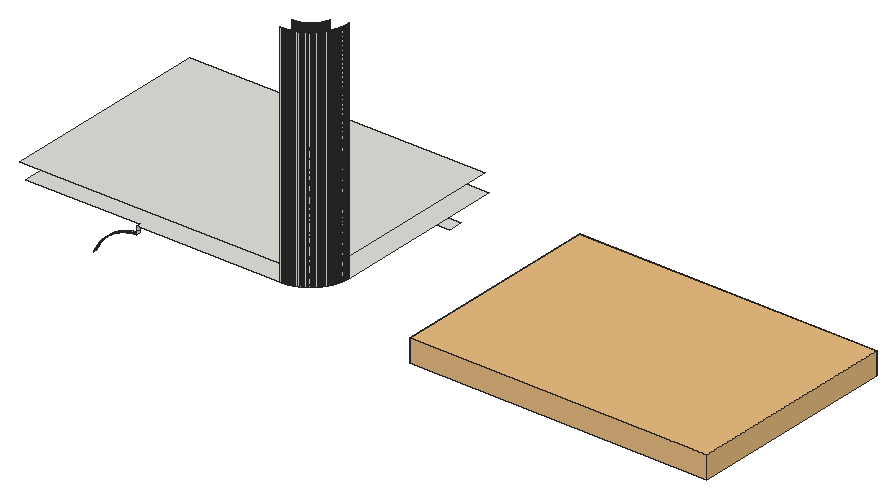
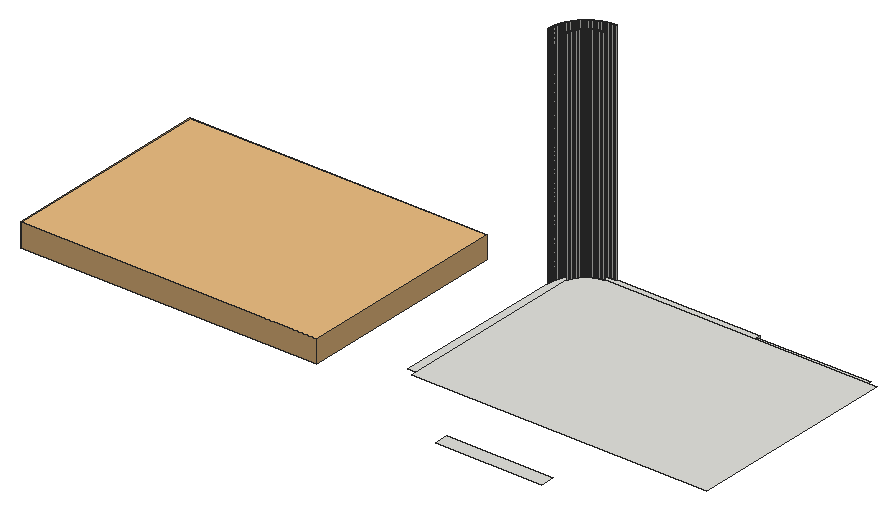
# SketchUp Ruby script. Lengths in inches.
U = 1.inch
M = Sketchup.active_model
def pt(a) = Geom::Point3d.new(a.map { |v| v * U })
def face(e, loops, mat)
  f = e.add_face(loops[0].map { |a| pt(a) })
  loops[1..].each { |l| e.add_face(l.map { |a| pt(a) }).erase! }
  f.material = f.back_material = mat if mat
  f
end
# faces: each face lists its corners as indices into pts; further lists are holes
def faces(e, pts, list, mat = nil) = list.each { |f| face(e, (f[0].is_a?(Array) ? f : [f]).map { |l| l.map { |i| pts[i] } }, mat) }
# xy, xz, yz: faces in a plane at the given z, y or x. An outline is a flat list of corners, or four numbers for a rectangle; further outlines are holes
def ring(l) = l.size == 4 ? [[l[0], l[1]], [l[2], l[1]], [l[2], l[3]], [l[0], l[3]]] : l.each_slice(2).to_a
def flat(e, list, mat, &to3) = list.each { |f| face(e, (f[0].is_a?(Array) ? f : [f]).map { |l| ring(l).map { |u, v| to3.(u, v) } }, mat) }
def xy(e, z, list, mat = nil) = flat(e, list, mat) { |x, y| [x, y, z] }
def xz(e, y, list, mat = nil) = flat(e, list, mat) { |x, z| [x, y, z] }
def yz(e, x, list, mat = nil) = flat(e, list, mat) { |y, z| [x, y, z] }
def lines(e, pts, list) = list.each { |a, b| e.add_line(pt(pts[a]), pt(pts[b])) }
# prism: a flat outline (further loops are holes) pulled along v
def prism(e, loops, v, mat = nil)
  f = face(e, loops, mat); d = Geom::Vector3d.new(v.map { |x| x * U })
  f.pushpull(f.normal.samedirection?(d) ? d.length : -d.length)
end
def box(e, o, s, mat = nil) = prism(e, [[o, [o[0] + s[0], o[1], o[2]], [o[0] + s[0], o[1] + s[1], o[2]], [o[0], o[1] + s[1], o[2]]]], [0, 0, s[2]], mat)
def at(x, y, z, deg = 0) = Geom::Transformation.translation(pt([x, y, z])) * Geom::Transformation.rotation(ORIGIN, Z_AXIS, deg.degrees)
def axes(o, x, y, z) = Geom::Transformation.new([*x, 0, *y, 0, *z, 0, *pt(o).to_a, 1])
def part(name) = M.definitions.add(name)
# library, detail: a bought-in or finely detailed component or shape, given as its bounding box
def library(name, o, s) = part(name).tap { |d| box(d.entities, o, s) }
def detail(e, o, s) = box(e.add_group.entities, o, s)
def put(e, d, t, mat = nil) = e.add_instance(d, t).tap { |i| i.material = mat if mat }
def group(e, t, mat = nil) = e.add_group.tap { |g| g.transformation = t; g.material = mat if mat }.entities
root = M.entities
c1 = library("Group\#26",[0,0,-14.0625],[184.56,132,14.0625])
xy(root,222,[[224.45,276,290.45,285]])
xy(root,251,[[201.56,144,201.56,146,131,146,131,276,314.45,276,314.45,167.375,314.43,167.06,314.42,166.75,314.4,166.43,314.38,166.12,314.35,165.81,314.32,165.49,314.29,165.18,314.21,164.56,314.16,164.25,314.11,163.9375,314.05,163.63,313.93,163.01,313.86,162.71,313.79,162.4,313.71,162.09,313.64,161.79,313.55,161.49,313.47,161.1875,313.375,160.89,313.28,160.59,313.08,159.99,312.97,159.7,312.86,159.4,312.74,159.11,312.625,158.82,312.5,158.53,312.38,158.24,312.25,157.95,312.12,157.67,311.84,157.11,311.69,156.83,311.55,156.55,311.39,156.28,311.24,156,310.92,155.46,310.75,155.2,310.58,154.93,310.41,154.67,310.05,154.15,309.87,153.9,309.68,153.64,309.3,153.14,309.1,152.9,308.91,152.66,308.7,152.42,308.5,152.18,308.29,151.94,308.08,151.71,307.86,151.48,307.64,151.26,307.42,151.03,307.2,150.8125,306.97,150.59,306.28,149.96,306.04,149.75,305.56,149.35,305.3125,149.15,304.8125,148.77,304.56,148.59,304.3,148.4,304.05,148.22,303.79,148.05,303.52,147.875,303.26,147.7,302.99,147.54,302.72,147.375,302.45,147.22,302.18,147.0625,301.91,146.91,301.63,146.76,300.79,146.34,300.5,146.21,300.22,146.08,299.93,145.95,299.35,145.71,299.05,145.6,298.76,145.49,298.46,145.38,298.17,145.28,297.57,145.08,296.97,144.9,296.67,144.82,296.36,144.74,296.06,144.67,295.75,144.59,295.44,144.53,295.14,144.46,294.83,144.4,293.9,144.25,293.59,144.21,293.27,144.17,292.96,144.13,292.65,144.1,292.34,144.08,292.02,144.05,291.71,144.03,291.4,144.02,291.08,144.01,290.77,144]])
xy(root,254.81,[[122,153,290.65,153,290.85,153.01,291.04,153.01,291.24,153.02,291.43,153.03,291.63,153.05,291.83,153.06,292.02,153.08,292.22,153.11,292.41,153.13,292.61,153.16,292.8,153.1875,292.99,153.22,293.1875,153.25,293.38,153.29,293.76,153.37,293.96,153.42,294.15,153.46,294.34,153.51,294.53,153.57,294.71,153.62,295.09,153.74,295.27,153.8,295.46,153.86,295.65,153.93,296.19,154.14,296.375,154.22,296.55,154.3,296.91,154.46,297.09,154.55,297.26,154.64,297.4375,154.73,297.61,154.82,297.78,154.91,298.29,155.21,298.46,155.32,298.62,155.42,298.79,155.53,299.11,155.75,299.27,155.87,299.43,155.98,299.58,156.1,299.74,156.22,299.89,156.34,300.04,156.47,300.2,156.6,300.34,156.72,300.49,156.85,300.64,156.99,300.78,157.12,301.2,157.54,301.33,157.68,301.47,157.82,301.6,157.97,301.73,158.11,301.99,158.41,302.11,158.5625,302.23,158.72,302.35,158.87,302.59,159.19,302.7,159.34,302.82,159.51,302.93,159.67,303.03,159.83,303.14,160,303.24,160.16,303.64,160.84,303.73,161.02,303.82,161.19,303.91,161.37,303.99,161.54,304.08,161.72,304.24,162.08,304.3125,162.26,304.39,162.44,304.53,162.81,304.59,162.99,304.66,163.18,304.72,163.37,304.78,163.55,304.84,163.74,304.99,164.31,305,164.34,305,285,122,285]])
xz(root,144,[[290.45,251,290.77,392.81]])
xz(root,153,[[290.45,254.81,290.65,392.81]])
xz(root,153.01,[[290.85,254.81,291.04,392.81]])
yz(root,201.56,[[144,248,146,251]])
yz(root,314.45,[[167.375,251,167.6875,392.81],[167.6875,251,168,392.81]])
p = [[175.15,144,227.49],[175.01,144,227.16],[175.01,146,227.16],[175.15,146,227.49],[175.3,144,227.82],[175.3,146,227.82],
  [175.44,144,228.14],[175.44,146,228.14],[175.59,144,228.47],[175.59,146,228.47],[175.74,144,228.79],[175.74,146,228.79],
  [175.9,144,229.11],[175.9,146,229.11],[176.06,144,229.42],[176.06,146,229.42],[176.22,144,229.74],[176.22,146,229.74],
  [176.39,144,230.05],[176.39,146,230.05],[176.5625,144,230.36],[176.5625,146,230.36],[176.74,144,230.67],[176.74,146,230.67],
  [176.92,144,230.98],[176.92,146,230.98],[177.1,144,231.29],[177.1,146,231.29],[177.28,144,231.59],[177.28,146,231.59],
  [177.47,144,231.89],[177.47,146,231.89],[177.66,144,232.19],[177.66,146,232.19],[177.86,144,232.49],[177.86,146,232.49],
  [178.06,144,232.78],[178.06,146,232.78],[178.26,144,233.07],[178.26,146,233.07],[178.47,144,233.36],[178.47,146,233.36],
  [178.68,144,233.65],[178.68,146,233.65],[178.89,144,233.9375],[178.89,146,233.9375],[179.1,144,234.22],[179.1,146,234.22],
  [179.32,144,234.5],[179.32,146,234.5],[179.55,144,234.78],[179.55,146,234.78],[179.77,144,235.05],[179.77,146,235.05],
  [180,144,235.33],[180,146,235.33],[180.23,144,235.6],[180.23,146,235.6],[180.46,144,235.86],[180.46,146,235.86],
  [180.7,144,236.13],[180.7,146,236.13],[180.94,144,236.39],[180.94,146,236.39],[181.1875,144,236.65],[181.1875,146,236.65],
  [181.43,144,236.9],[181.43,146,236.9],[181.68,144,237.16],[181.68,146,237.16],[181.93,144,237.41],[181.93,146,237.41],
  [182.19,144,237.66],[182.19,146,237.66],[182.45,144,237.9],[182.45,146,237.9],[182.71,144,238.14],[182.71,146,238.14],
  [182.97,144,238.38],[182.97,146,238.38],[183.24,144,238.62],[183.24,146,238.62],[183.51,144,238.85],[183.51,146,238.85],
  [183.78,144,239.08],[183.78,146,239.08],[184.05,144,239.31],[184.05,146,239.31],[184.33,144,239.53],[184.33,146,239.53],
  [184.61,144,239.75],[184.61,146,239.75],[184.89,144,239.97],[184.89,146,239.97],[185.18,144,240.18],[185.18,146,240.18],
  [185.46,144,240.39],[185.46,146,240.39],[185.75,144,240.6],[185.75,146,240.6],[186.04,144,240.8],[186.04,146,240.8],
  [186.34,144,241],[186.34,146,241],[186.63,144,241.2],[186.63,146,241.2],[186.93,144,241.39],[186.93,146,241.39],
  [187.23,144,241.58],[187.23,146,241.58],[187.54,144,241.77],[187.54,146,241.77],[187.84,144,241.95],[187.84,146,241.95],
  [188.15,144,242.13],[188.15,146,242.13],[188.46,144,242.31],[188.46,146,242.31],[188.77,144,242.48],[188.77,146,242.48],
  [189.08,144,242.65],[189.08,146,242.65],[189.4,144,242.8125],[189.4,146,242.8125],[189.71,144,242.97],[189.71,146,242.97],
  [190.03,144,243.13],[190.03,146,243.13],[190.35,144,243.29],[190.35,146,243.29],[190.67,144,243.4375],[190.67,146,243.4375],
  [191,144,243.58],[191,146,243.58],[191.32,144,243.73],[191.32,146,243.73],[191.65,144,243.87],[191.65,146,243.87],
  [191.98,144,244],[191.98,146,244],[192.31,144,244.13],[192.31,146,244.13],[192.64,144,244.26],[192.64,146,244.26],
  [192.97,144,244.39],[192.97,146,244.39],[193.31,144,244.51],[193.31,146,244.51],[193.64,144,244.625],[193.64,146,244.625],
  [193.98,144,244.74],[193.98,146,244.74],[194.32,144,244.85],[194.32,146,244.85],[194.66,144,244.95],[194.66,146,244.95],
  [195,144,245.05],[195,146,245.05],[195.34,144,245.15],[195.34,146,245.15],[195.68,144,245.24],[195.68,146,245.24],
  [196.03,144,245.33],[196.03,146,245.33],[196.375,144,245.42],[196.375,146,245.42],[196.72,144,245.5],[196.72,146,245.5],
  [197.07,144,245.58],[197.07,146,245.58],[197.42,144,245.65],[197.42,146,245.65],[197.76,144,245.72],[197.76,146,245.72],
  [198.11,144,245.78],[198.11,146,245.78],[198.46,144,245.85],[198.46,146,245.85],[198.81,144,245.9],[198.81,146,245.9],
  [199.17,144,245.96],[199.17,146,245.96],[199.52,144,246.01],[199.52,146,246.01],[199.87,144,246.05],[199.87,146,246.05],
  [200.22,144,246.09],[200.22,146,246.09],[200.58,144,246.13],[200.58,146,246.13],[200.93,144,246.16],[200.93,146,246.16],
  [201.29,144,246.19],[201.29,146,246.19],[201.64,144,246.22],[201.64,146,246.22],[201.56,144,248],[201.56,146,248],
  [290.77,144,392.81],[290.77,144,251],[291.08,144.01,251],[291.08,144.01,392.81],[291.4,144.02,251],[291.4,144.02,392.81],
  [291.71,144.03,251],[291.71,144.03,392.81],[292.02,144.05,251],[292.02,144.05,392.81],[292.34,144.08,251],[292.34,144.08,392.81],
  [292.65,144.1,251],[292.65,144.1,392.81],[292.96,144.13,251],[292.96,144.13,392.81],[293.27,144.17,251],[293.27,144.17,392.81],
  [293.59,144.21,251],[293.59,144.21,392.81],[293.9,144.25,251],[293.9,144.25,392.81],[294.21,144.3,251],[294.21,144.3,392.81],
  [294.52,144.35,251],[294.52,144.35,392.81],[294.83,144.4,251],[294.83,144.4,392.81],[295.14,144.46,251],[295.14,144.46,392.81],
  [295.44,144.53,251],[295.44,144.53,392.81],[295.75,144.59,251],[295.75,144.59,392.81],[296.06,144.67,251],[296.06,144.67,392.81],
  [296.36,144.74,251],[296.36,144.74,392.81],[296.67,144.82,251],[296.67,144.82,392.81],[296.97,144.9,251],[296.97,144.9,392.81],
  [297.27,144.99,251],[297.27,144.99,392.81],[297.57,145.08,251],[297.57,145.08,392.81],[297.87,145.18,251],[297.87,145.18,392.81],
  [298.17,145.28,251],[298.17,145.28,392.81],[298.46,145.38,251],[298.46,145.38,392.81],[298.76,145.49,251],[298.76,145.49,392.81],
  [299.05,145.6,251],[299.05,145.6,392.81],[299.35,145.71,251],[299.35,145.71,392.81],[299.64,145.83,251],[299.64,145.83,392.81],
  [299.93,145.95,251],[299.93,145.95,392.81],[300.22,146.08,251],[300.22,146.08,392.81],[300.5,146.21,251],[300.5,146.21,392.81],
  [300.79,146.34,251],[300.79,146.34,392.81],[301.07,146.48,251],[301.07,146.48,392.81],[301.35,146.62,251],[301.35,146.62,392.81],
  [301.63,146.76,251],[301.63,146.76,392.81],[301.91,146.91,251],[301.91,146.91,392.81],[302.18,147.0625,251],[302.18,147.0625,392.81],
  [302.45,147.22,251],[302.45,147.22,392.81],[302.72,147.375,251],[302.72,147.375,392.81],[302.99,147.54,251],[302.99,147.54,392.81],
  [303.26,147.7,251],[303.26,147.7,392.81],[303.52,147.875,251],[303.52,147.875,392.81],[303.79,148.05,251],[303.79,148.05,392.81],
  [304.05,148.22,251],[304.05,148.22,392.81],[304.3,148.4,251],[304.3,148.4,392.81],[304.56,148.59,251],[304.56,148.59,392.81],
  [304.8125,148.77,251],[304.8125,148.77,392.81],[305.0625,148.96,251],[305.0625,148.96,392.81],[305.3125,149.15,251],[305.3125,149.15,392.81],
  [305.56,149.35,251],[305.56,149.35,392.81],[305.8,149.55,251],[305.8,149.55,392.81],[306.04,149.75,251],[306.04,149.75,392.81],
  [306.28,149.96,251],[306.28,149.96,392.81],[306.51,150.17,251],[306.51,150.17,392.81],[306.74,150.38,251],[306.74,150.38,392.81],
  [306.97,150.59,251],[306.97,150.59,392.81],[307.2,150.8125,251],[307.2,150.8125,392.81],[307.42,151.03,251],[307.42,151.03,392.81],
  [307.64,151.26,251],[307.64,151.26,392.81],[307.86,151.48,251],[307.86,151.48,392.81],[308.08,151.71,251],[308.08,151.71,392.81],
  [308.29,151.94,251],[308.29,151.94,392.81],[308.5,152.18,251],[308.5,152.18,392.81],[308.7,152.42,251],[308.7,152.42,392.81],
  [308.91,152.66,251],[308.91,152.66,392.81],[309.1,152.9,251],[309.1,152.9,392.81],[309.3,153.14,251],[309.3,153.14,392.81],
  [309.49,153.39,251],[309.49,153.39,392.81],[309.68,153.64,251],[309.68,153.64,392.81],[309.87,153.9,251],[309.87,153.9,392.81],
  [310.05,154.15,251],[310.05,154.15,392.81],[310.23,154.41,251],[310.23,154.41,392.81],[310.41,154.67,251],[310.41,154.67,392.81],
  [310.58,154.93,251],[310.58,154.93,392.81],[310.75,155.2,251],[310.75,155.2,392.81],[310.92,155.46,251],[310.92,155.46,392.81],
  [311.08,155.73,251],[311.08,155.73,392.81],[311.24,156,251],[311.24,156,392.81],[311.39,156.28,251],[311.39,156.28,392.81],
  [311.55,156.55,251],[311.55,156.55,392.81],[311.69,156.83,251],[311.69,156.83,392.81],[311.84,157.11,251],[311.84,157.11,392.81],
  [311.98,157.39,251],[311.98,157.39,392.81],[312.12,157.67,251],[312.12,157.67,392.81],[312.25,157.95,251],[312.25,157.95,392.81],
  [312.38,158.24,251],[312.38,158.24,392.81],[312.5,158.53,251],[312.5,158.53,392.81],[312.625,158.82,251],[312.625,158.82,392.81],
  [312.74,159.11,251],[312.74,159.11,392.81],[312.86,159.4,251],[312.86,159.4,392.81],[312.97,159.7,251],[312.97,159.7,392.81],
  [313.08,159.99,251],[313.08,159.99,392.81],[313.18,160.29,251],[313.18,160.29,392.81],[313.28,160.59,251],[313.28,160.59,392.81],
  [313.375,160.89,251],[313.375,160.89,392.81],[313.47,161.1875,251],[313.47,161.1875,392.81],[313.55,161.49,251],[313.55,161.49,392.81],
  [313.64,161.79,251],[313.64,161.79,392.81],[313.71,162.09,251],[313.71,162.09,392.81],[313.79,162.4,251],[313.79,162.4,392.81],
  [313.86,162.71,251],[313.86,162.71,392.81],[313.93,163.01,251],[313.93,163.01,392.81],[313.99,163.32,251],[313.99,163.32,392.81],
  [314.05,163.63,251],[314.05,163.63,392.81],[314.11,163.9375,251],[314.11,163.9375,392.81],[314.16,164.25,251],[314.16,164.25,392.81],
  [314.21,164.56,251],[314.21,164.56,392.81],[314.25,164.87,251],[314.25,164.87,392.81],[314.29,165.18,251],[314.29,165.18,392.81],
  [314.32,165.49,251],[314.32,165.49,392.81],[314.35,165.81,251],[314.35,165.81,392.81],[314.38,166.12,251],[314.38,166.12,392.81],
  [314.4,166.43,251],[314.4,166.43,392.81],[314.42,166.75,251],[314.42,166.75,392.81],[314.43,167.06,251],[314.43,167.06,392.81],
  [314.45,167.375,251],[314.45,167.375,392.81],[290.65,153,392.81],[290.85,153.01,392.81],[290.85,153.01,254.81],[290.65,153,254.81],
  [291.04,153.01,392.81],[291.24,153.02,392.81],[291.24,153.02,254.81],[291.04,153.01,254.81],[291.43,153.03,392.81],[291.43,153.03,254.81],
  [291.63,153.05,392.81],[291.63,153.05,254.81],[291.83,153.06,392.81],[291.83,153.06,254.81],[292.02,153.08,392.81],[292.02,153.08,254.81],
  [292.22,153.11,392.81],[292.22,153.11,254.81],[292.41,153.13,392.81],[292.41,153.13,254.81],[292.61,153.16,392.81],[292.61,153.16,254.81],
  [292.8,153.1875,392.81],[292.8,153.1875,254.81],[292.99,153.22,392.81],[292.99,153.22,254.81],[293.1875,153.25,392.81],[293.1875,153.25,254.81],
  [293.38,153.29,392.81],[293.38,153.29,254.81],[293.57,153.33,392.81],[293.57,153.33,254.81],[293.76,153.37,392.81],[293.76,153.37,254.81],
  [293.96,153.42,392.81],[293.96,153.42,254.81],[294.15,153.46,392.81],[294.15,153.46,254.81],[294.34,153.51,392.81],[294.34,153.51,254.81],
  [294.53,153.57,392.81],[294.53,153.57,254.81],[294.71,153.62,392.81],[294.71,153.62,254.81],[294.9,153.68,392.81],[294.9,153.68,254.81],
  [295.09,153.74,392.81],[295.09,153.74,254.81],[295.27,153.8,392.81],[295.27,153.8,254.81],[295.46,153.86,392.81],[295.46,153.86,254.81],
  [295.65,153.93,392.81],[295.65,153.93,254.81],[295.83,154,392.81],[295.83,154,254.81],[296.01,154.07,392.81],[296.01,154.07,254.81],
  [296.19,154.14,392.81],[296.19,154.14,254.81],[296.375,154.22,392.81],[296.375,154.22,254.81],[296.55,154.3,392.81],[296.55,154.3,254.81],
  [296.73,154.38,392.81],[296.73,154.38,254.81],[296.91,154.46,392.81],[296.91,154.46,254.81],[297.09,154.55,392.81],[297.09,154.55,254.81],
  [297.26,154.64,392.81],[297.26,154.64,254.81],[297.4375,154.73,392.81],[297.4375,154.73,254.81],[297.61,154.82,392.81],[297.61,154.82,254.81],
  [297.78,154.91,392.81],[297.78,154.91,254.81],[297.95,155.01,392.81],[297.95,155.01,254.81],[298.12,155.11,392.81],[298.12,155.11,254.81],
  [298.29,155.21,392.81],[298.29,155.21,254.81],[298.46,155.32,392.81],[298.46,155.32,254.81],[298.62,155.42,392.81],[298.62,155.42,254.81],
  [298.79,155.53,392.81],[298.79,155.53,254.81],[298.95,155.64,392.81],[298.95,155.64,254.81],[299.11,155.75,392.81],[299.11,155.75,254.81],
  [299.27,155.87,392.81],[299.27,155.87,254.81],[299.43,155.98,392.81],[299.43,155.98,254.81],[299.58,156.1,392.81],[299.58,156.1,254.81],
  [299.74,156.22,392.81],[299.74,156.22,254.81],[299.89,156.34,392.81],[299.89,156.34,254.81],[300.04,156.47,392.81],[300.04,156.47,254.81],
  [300.2,156.6,392.81],[300.2,156.6,254.81],[300.34,156.72,392.81],[300.34,156.72,254.81],[300.49,156.85,392.81],[300.49,156.85,254.81],
  [300.64,156.99,392.81],[300.64,156.99,254.81],[300.78,157.12,392.81],[300.78,157.12,254.81],[300.92,157.26,392.81],[300.92,157.26,254.81],
  [301.06,157.4,392.81],[301.06,157.4,254.81],[301.2,157.54,392.81],[301.2,157.54,254.81],[301.33,157.68,392.81],[301.33,157.68,254.81],
  [301.47,157.82,392.81],[301.47,157.82,254.81],[301.6,157.97,392.81],[301.6,157.97,254.81],[301.73,158.11,392.81],[301.73,158.11,254.81],
  [301.86,158.26,392.81],[301.86,158.26,254.81],[301.99,158.41,392.81],[301.99,158.41,254.81],[302.11,158.5625,392.81],[302.11,158.5625,254.81],
  [302.23,158.72,392.81],[302.23,158.72,254.81],[302.35,158.87,392.81],[302.35,158.87,254.81],[302.47,159.03,392.81],[302.47,159.03,254.81],
  [302.59,159.19,392.81],[302.59,159.19,254.81],[302.7,159.34,392.81],[302.7,159.34,254.81],[302.82,159.51,392.81],[302.82,159.51,254.81],
  [302.93,159.67,392.81],[302.93,159.67,254.81],[303.03,159.83,392.81],[303.03,159.83,254.81],[303.14,160,392.81],[303.14,160,254.81],
  [303.24,160.16,392.81],[303.24,160.16,254.81],[303.34,160.33,392.81],[303.34,160.33,254.81],[303.44,160.5,392.81],[303.44,160.5,254.81],
  [303.54,160.67,392.81],[303.54,160.67,254.81],[303.64,160.84,392.81],[303.64,160.84,254.81],[303.73,161.02,392.81],[303.73,161.02,254.81],
  [303.82,161.19,392.81],[303.82,161.19,254.81],[303.91,161.37,392.81],[303.91,161.37,254.81],[303.99,161.54,392.81],[303.99,161.54,254.81],
  [304.08,161.72,392.81],[304.08,161.72,254.81],[304.16,161.9,392.81],[304.16,161.9,254.81],[304.24,162.08,392.81],[304.24,162.08,254.81],
  [304.3125,162.26,392.81],[304.3125,162.26,254.81],[304.39,162.44,392.81],[304.39,162.44,254.81],[304.46,162.625,392.81],[304.46,162.625,254.81],
  [304.53,162.81,392.81],[304.53,162.81,254.81],[304.59,162.99,392.81],[304.59,162.99,254.81],[304.66,163.18,392.81],[304.66,163.18,254.81],
  [304.72,163.37,392.81],[304.72,163.37,254.81],[304.78,163.55,392.81],[304.78,163.55,254.81],[304.84,163.74,392.81],[304.84,163.74,254.81],
  [304.89,163.93,392.81],[304.89,163.93,254.81],[304.94,164.12,392.81],[304.94,164.12,254.81],[304.99,164.31,392.81],[304.99,164.31,254.81],
  [305,164.34,392.81],[305,164.34,254.81],[131,146,248],[131,144,248],[305,153,254.81],[290.45,153,254.81],
  [305,153,392.81]]
faces(root,p,[[0,1,2,3],[4,0,3,5],[6,4,5,7],[8,6,7,9],[10,8,9,11],[12,10,11,13],[14,12,13,15],[16,14,15,17],
  [18,16,17,19],[20,18,19,21],[22,20,21,23],[24,22,23,25],[26,24,25,27],[28,26,27,29],[30,28,29,31],[32,30,31,33],
  [34,32,33,35],[36,34,35,37],[38,36,37,39],[40,38,39,41],[42,40,41,43],[44,42,43,45],[46,44,45,47],[48,46,47,49],
  [50,48,49,51],[52,50,51,53],[54,52,53,55],[56,54,55,57],[58,56,57,59],[60,58,59,61],[62,60,61,63],[64,62,63,65],
  [66,64,65,67],[68,66,67,69],[70,68,69,71],[72,70,71,73],[74,72,73,75],[76,74,75,77],[78,76,77,79],[80,78,79,81],
  [82,80,81,83],[84,82,83,85],[86,84,85,87],[88,86,87,89],[90,88,89,91],[92,90,91,93],[94,92,93,95],[96,94,95,97],
  [98,96,97,99],[100,98,99,101],[102,100,101,103],[104,102,103,105],[106,104,105,107],[108,106,107,109],[110,108,109,111],[112,110,111,113],
  [114,112,113,115],[116,114,115,117],[118,116,117,119],[120,118,119,121],[122,120,121,123],[124,122,123,125],[126,124,125,127],[128,126,127,129],
  [130,128,129,131],[132,130,131,133],[134,132,133,135],[136,134,135,137],[138,136,137,139],[140,138,139,141],[142,140,141,143],[144,142,143,145],
  [146,144,145,147],[148,146,147,149],[150,148,149,151],[152,150,151,153],[154,152,153,155],[156,154,155,157],[158,156,157,159],[160,158,159,161],
  [162,160,161,163],[164,162,163,165],[166,164,165,167],[168,166,167,169],[170,168,169,171],[172,170,171,173],[174,172,173,175],[176,174,175,177],
  [178,176,177,179],[180,178,179,181],[182,180,181,183],[184,182,183,185],[186,184,185,187],[188,186,187,189],[190,188,189,191],[192,190,191,193],
  [194,192,193,195],[196,194,195,197],[198,199,200,201],[201,200,202,203],[203,202,204,205],[205,204,206,207],[207,206,208,209],[209,208,210,211],
  [211,210,212,213],[213,212,214,215],[215,214,216,217],[217,216,218,219],[219,218,220,221],[221,220,222,223],[223,222,224,225],[225,224,226,227],
  [227,226,228,229],[229,228,230,231],[231,230,232,233],[233,232,234,235],[235,234,236,237],[237,236,238,239],[239,238,240,241],[241,240,242,243],
  [243,242,244,245],[245,244,246,247],[247,246,248,249],[249,248,250,251],[251,250,252,253],[253,252,254,255],[255,254,256,257],[257,256,258,259],
  [259,258,260,261],[261,260,262,263],[263,262,264,265],[265,264,266,267],[267,266,268,269],[269,268,270,271],[271,270,272,273],[273,272,274,275],
  [275,274,276,277],[277,276,278,279],[279,278,280,281],[281,280,282,283],[283,282,284,285],[285,284,286,287],[287,286,288,289],[289,288,290,291],
  [291,290,292,293],[293,292,294,295],[295,294,296,297],[297,296,298,299],[299,298,300,301],[301,300,302,303],[303,302,304,305],[305,304,306,307],
  [307,306,308,309],[309,308,310,311],[311,310,312,313],[313,312,314,315],[315,314,316,317],[317,316,318,319],[319,318,320,321],[321,320,322,323],
  [323,322,324,325],[325,324,326,327],[327,326,328,329],[329,328,330,331],[331,330,332,333],[333,332,334,335],[335,334,336,337],[337,336,338,339],
  [339,338,340,341],[341,340,342,343],[343,342,344,345],[345,344,346,347],[347,346,348,349],[349,348,350,351],[351,350,352,353],[353,352,354,355],
  [355,354,356,357],[357,356,358,359],[359,358,360,361],[361,360,362,363],[363,362,364,365],[365,364,366,367],[367,366,368,369],[369,368,370,371],
  [371,370,372,373],[373,372,374,375],[375,374,376,377],[377,376,378,379],[379,378,380,381],[381,380,382,383],[383,382,384,385],[385,384,386,387],
  [387,386,388,389],[389,388,390,391],[391,390,392,393],[393,392,394,395],[395,394,396,397],[397,396,398,399],[399,398,400,401],[401,400,402,403],
  [403,402,404,405],[405,404,406,407],[407,406,408,409],[409,408,410,411],[411,410,412,413],[413,412,414,415],[415,414,416,417],[417,416,418,419],
  [419,418,420,421],[421,420,422,423],[423,422,424,425],[425,424,426,427],[427,426,428,429],[429,428,430,431],[431,430,432,433],[434,435,436,437],
  [438,439,440,441],[439,442,443,440],[442,444,445,443],[444,446,447,445],[446,448,449,447],[448,450,451,449],[450,452,453,451],[452,454,455,453],
  [454,456,457,455],[456,458,459,457],[458,460,461,459],[460,462,463,461],[462,464,465,463],[464,466,467,465],[466,468,469,467],[468,470,471,469],
  [470,472,473,471],[472,474,475,473],[474,476,477,475],[476,478,479,477],[478,480,481,479],[480,482,483,481],[482,484,485,483],[484,486,487,485],
  [486,488,489,487],[488,490,491,489],[490,492,493,491],[492,494,495,493],[494,496,497,495],[496,498,499,497],[498,500,501,499],[500,502,503,501],
  [502,504,505,503],[504,506,507,505],[506,508,509,507],[508,510,511,509],[510,512,513,511],[512,514,515,513],[514,516,517,515],[516,518,519,517],
  [518,520,521,519],[520,522,523,521],[522,524,525,523],[524,526,527,525],[526,528,529,527],[528,530,531,529],[530,532,533,531],[532,534,535,533],
  [534,536,537,535],[536,538,539,537],[538,540,541,539],[540,542,543,541],[542,544,545,543],[544,546,547,545],[546,548,549,547],[548,550,551,549],
  [550,552,553,551],[552,554,555,553],[554,556,557,555],[556,558,559,557],[558,560,561,559],[560,562,563,561],[562,564,565,563],[564,566,567,565],
  [566,568,569,567],[568,570,571,569],[570,572,573,571],[572,574,575,573],[574,576,577,575],[576,578,579,577],[578,580,581,579],[580,582,583,581],
  [582,584,585,583],[584,586,587,585],[586,588,589,587],[588,590,591,589],[590,592,593,591],[592,594,595,593],[594,596,597,595],[596,598,599,597],
  [598,600,601,599],[600,602,603,601],[602,604,605,603],[604,606,607,605],[606,608,609,607],[608,610,611,609],[610,612,613,611],[612,614,615,613],
  [614,616,617,615],[616,618,619,617],[618,620,621,619],[620,622,623,621],[622,624,625,623],[624,626,627,625],[626,628,629,627],[628,630,631,629],
  [630,632,633,631],[632,634,635,633],[634,636,637,635]])
lines(root,p,[[638,639],[640,641],[642,640],[637,640]])
put(root,c1,at(371,144,248))
